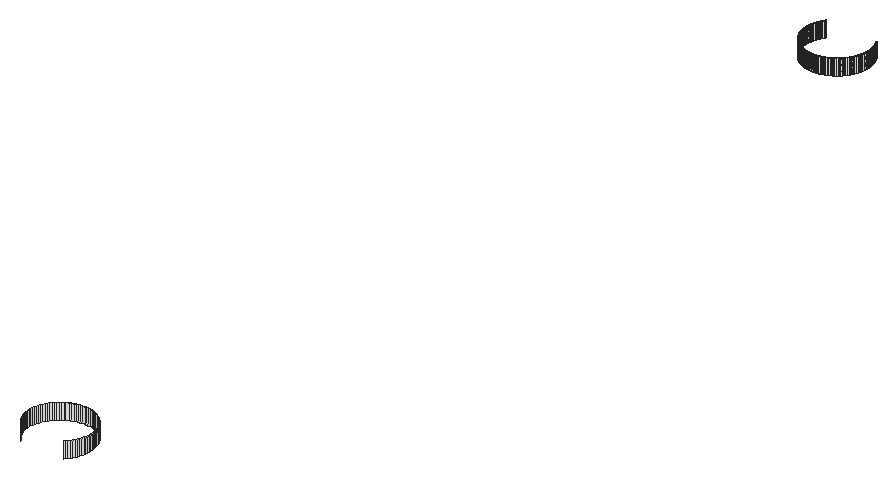
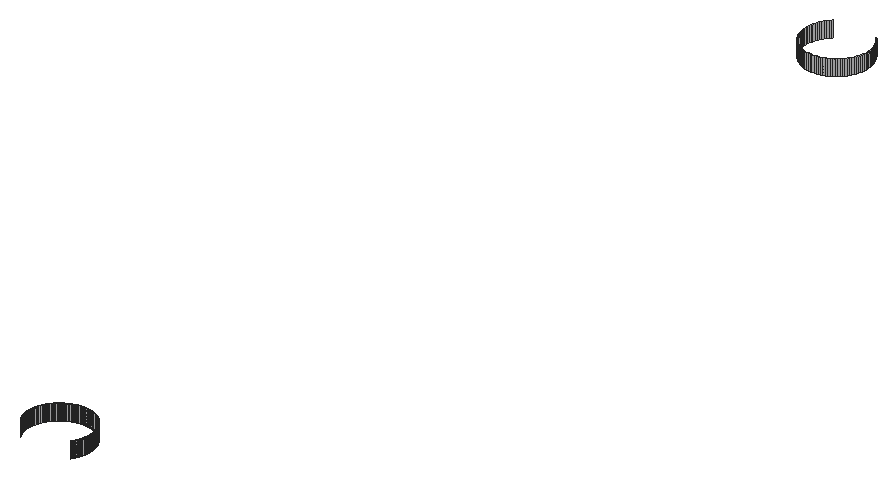
# SketchUp Ruby script. Lengths in inches.
U = 1.inch
M = Sketchup.active_model
def pt(a) = Geom::Point3d.new(a.map { |v| v * U })
def face(e, loops, mat)
  f = e.add_face(loops[0].map { |a| pt(a) })
  loops[1..].each { |l| e.add_face(l.map { |a| pt(a) }).erase! }
  f.material = f.back_material = mat if mat
  f
end
# faces: each face lists its corners as indices into pts; further lists are holes
def faces(e, pts, list, mat = nil) = list.each { |f| face(e, (f[0].is_a?(Array) ? f : [f]).map { |l| l.map { |i| pts[i] } }, mat) }
# xy, xz, yz: faces in a plane at the given z, y or x. An outline is a flat list of corners, or four numbers for a rectangle; further outlines are holes
def ring(l) = l.size == 4 ? [[l[0], l[1]], [l[2], l[1]], [l[2], l[3]], [l[0], l[3]]] : l.each_slice(2).to_a
def flat(e, list, mat, &to3) = list.each { |f| face(e, (f[0].is_a?(Array) ? f : [f]).map { |l| ring(l).map { |u, v| to3.(u, v) } }, mat) }
def xy(e, z, list, mat = nil) = flat(e, list, mat) { |x, y| [x, y, z] }
def xz(e, y, list, mat = nil) = flat(e, list, mat) { |x, z| [x, y, z] }
def yz(e, x, list, mat = nil) = flat(e, list, mat) { |y, z| [x, y, z] }
def lines(e, pts, list) = list.each { |a, b| e.add_line(pt(pts[a]), pt(pts[b])) }
# prism: a flat outline (further loops are holes) pulled along v
def prism(e, loops, v, mat = nil)
  f = face(e, loops, mat); d = Geom::Vector3d.new(v.map { |x| x * U })
  f.pushpull(f.normal.samedirection?(d) ? d.length : -d.length)
end
def box(e, o, s, mat = nil) = prism(e, [[o, [o[0] + s[0], o[1], o[2]], [o[0] + s[0], o[1] + s[1], o[2]], [o[0], o[1] + s[1], o[2]]]], [0, 0, s[2]], mat)
def at(x, y, z, deg = 0) = Geom::Transformation.translation(pt([x, y, z])) * Geom::Transformation.rotation(ORIGIN, Z_AXIS, deg.degrees)
def axes(o, x, y, z) = Geom::Transformation.new([*x, 0, *y, 0, *z, 0, *pt(o).to_a, 1])
def part(name) = M.definitions.add(name)
# library, detail: a bought-in or finely detailed component or shape, given as its bounding box
def library(name, o, s) = part(name).tap { |d| box(d.entities, o, s) }
def detail(e, o, s) = box(e.add_group.entities, o, s)
def put(e, d, t, mat = nil) = e.add_instance(d, t).tap { |i| i.material = mat if mat }
def group(e, t, mat = nil) = e.add_group.tap { |g| g.transformation = t; g.material = mat if mat }.entities
root = M.entities
M.materials.add("[Quartz Light Grey]").color = [251, 251, 252]
xz(root,170.71,[[32.98,111.81,33.1,112.81]],"[Quartz Light Grey]")
xz(root,222.0625,[[38.98,111.81,39,112.81],[39,111.81,39.02,112.81]],"[Quartz Light Grey]")
xz(root,222.07,[[38.8125,111.81,38.85,112.81],[38.85,111.81,38.875,112.81],[38.875,111.81,38.9,112.81],[39.1,111.81,39.125,112.81],[39.125,111.81,39.15,112.81],
  [39.15,111.81,39.1875,112.81]],"[Quartz Light Grey]")
xz(root,222.08,[[38.73,111.81,38.75,112.81],[38.75,111.81,38.77,112.81],[39.23,111.81,39.25,112.81],[39.25,111.81,39.27,112.81]],"[Quartz Light Grey]")
xz(root,222.09,[[38.65,111.81,38.6875,112.81],[39.3125,111.81,39.35,112.81]],"[Quartz Light Grey]")
xz(root,222.1,[[38.6,111.81,38.625,112.81],[39.375,111.81,39.4,112.81]],"[Quartz Light Grey]")
xz(root,222.2,[[38.26,111.81,38.28,112.81],[39.72,111.81,39.74,112.81]],"[Quartz Light Grey]")
yz(root,31,[[168.6875,111.81,168.8125,112.81]],"[Quartz Light Grey]")
yz(root,35,[[168.6,111.81,168.73,112.81]],"[Quartz Light Grey]")
yz(root,37,[[223.9375,111.81,223.96,112.81],[223.96,111.81,224,112.81],[224,111.81,224.04,112.81],[224.04,111.81,224.0625,112.81],[224.0625,111.81,224.08,112.81],
  [224.08,111.81,224.125,112.81],[224.125,111.81,224.17,112.81],[224.17,111.81,224.1875,112.81]],"[Quartz Light Grey]")
yz(root,37.01,[[223.83,111.81,223.875,112.81],[223.875,111.81,223.92,112.81],[224.21,111.81,224.25,112.81],[224.25,111.81,224.29,112.81]],"[Quartz Light Grey]")
yz(root,37.02,[[223.79,111.81,223.8125,112.81],[224.3125,111.81,224.33,112.81]],"[Quartz Light Grey]")
yz(root,37.03,[[223.71,111.81,223.75,112.81],[224.375,111.81,224.42,112.81]],"[Quartz Light Grey]")
yz(root,37.04,[[223.67,111.81,223.6875,112.81],[224.4375,111.81,224.46,112.81]],"[Quartz Light Grey]")
yz(root,37.1,[[223.42,111.81,223.44,112.81],[224.68,111.81,224.7,112.81]],"[Quartz Light Grey]")
yz(root,40.9,[[223.42,111.81,223.44,112.81],[224.68,111.81,224.7,112.81]],"[Quartz Light Grey]")
yz(root,40.96,[[223.67,111.81,223.6875,112.81],[224.4375,111.81,224.46,112.81]],"[Quartz Light Grey]")
yz(root,40.97,[[223.71,111.81,223.75,112.81],[224.375,111.81,224.42,112.81]],"[Quartz Light Grey]")
yz(root,40.98,[[223.79,111.81,223.8125,112.81],[224.3125,111.81,224.33,112.81]],"[Quartz Light Grey]")
yz(root,40.99,[[223.83,111.81,223.875,112.81],[223.875,111.81,223.92,112.81],[224.21,111.81,224.25,112.81],[224.25,111.81,224.29,112.81]],"[Quartz Light Grey]")
yz(root,41,[[223.9375,111.81,223.96,112.81],[223.96,111.81,224,112.81],[224,111.81,224.04,112.81],[224.04,111.81,224.0625,112.81],[224.0625,111.81,224.08,112.81],
  [224.08,111.81,224.125,112.81],[224.125,111.81,224.17,112.81],[224.17,111.81,224.1875,112.81]],"[Quartz Light Grey]")
p = [[31.56,167.32,111.81],[31.47,167.42,111.81],[31.47,167.42,112.81],[31.56,167.32,112.81],[34.47,167.36,111.81],[34.38,167.27,111.81],
  [34.38,167.27,112.81],[34.47,167.36,112.81],[31.39,167.52,111.81],[31.39,167.52,112.81],[34.55,167.45,111.81],[34.55,167.45,112.81],
  [31.32,167.62,111.81],[31.32,167.62,112.81],[34.63,167.55,111.81],[34.63,167.55,112.81],[31.26,167.73,111.81],[31.26,167.73,112.81],
  [34.7,167.66,111.81],[34.7,167.66,112.81],[31.2,167.84,111.81],[31.2,167.84,112.81],[34.76,167.76,111.81],[34.76,167.76,112.81],
  [31.15,167.95,111.81],[31.15,167.95,112.81],[34.82,167.875,111.81],[34.82,167.875,112.81],[34.87,167.99,111.81],[34.87,167.99,112.81],
  [31.1,168.07,111.81],[31.1,168.07,112.81],[34.91,168.11,111.81],[34.91,168.11,112.81],[31.07,168.19,111.81],[31.07,168.19,112.81],
  [34.94,168.23,111.81],[34.94,168.23,112.81],[31.04,168.3125,111.81],[31.04,168.3125,112.81],[34.97,168.35,111.81],[34.97,168.35,112.81],
  [31.02,168.4375,111.81],[31.02,168.4375,112.81],[31.01,168.5625,111.81],[31.01,168.5625,112.81],[34.99,168.48,111.81],[34.99,168.48,112.81],
  [35,168.6,111.81],[35,168.6,112.81],[31,168.6875,111.81],[31,168.6875,112.81],[34.99,168.86,111.81],[35,168.73,111.81],
  [35,168.73,112.81],[34.99,168.86,112.81],[31,168.8125,111.81],[31.01,168.9375,111.81],[31.01,168.9375,112.81],[31,168.8125,112.81],
  [31.03,169.0625,111.81],[31.03,169.0625,112.81],[34.98,168.98,111.81],[34.98,168.98,112.81],[34.96,169.1,111.81],[34.96,169.1,112.81],
  [31.06,169.19,111.81],[31.06,169.19,112.81],[34.93,169.23,111.81],[34.93,169.23,112.81],[31.09,169.31,111.81],[31.09,169.31,112.81],
  [34.9,169.35,111.81],[34.9,169.35,112.81],[31.13,169.42,111.81],[31.13,169.42,112.81],[34.85,169.46,111.81],[34.85,169.46,112.81],
  [31.18,169.54,111.81],[31.18,169.54,112.81],[31.24,169.65,111.81],[31.24,169.65,112.81],[34.8,169.58,111.81],[34.8,169.58,112.81],
  [34.74,169.69,111.81],[34.74,169.69,112.81],[31.3,169.76,111.81],[31.3,169.76,112.81],[34.68,169.8,111.81],[34.68,169.8,112.81],
  [31.37,169.87,111.81],[31.37,169.87,112.81],[34.61,169.9,111.81],[34.61,169.9,112.81],[31.45,169.97,111.81],[31.45,169.97,112.81],
  [34.53,170,111.81],[34.53,170,112.81],[31.53,170.0625,111.81],[31.53,170.0625,112.81],[34.44,170.09,111.81],[34.44,170.09,112.81],
  [31.62,170.15,111.81],[31.62,170.15,112.81],[34.35,170.18,111.81],[34.35,170.18,112.81],[31.71,170.24,111.81],[31.71,170.24,112.81],
  [31.81,170.3125,111.81],[31.81,170.3125,112.81],[34.26,170.26,111.81],[34.26,170.26,112.81],[31.91,170.39,111.81],[31.91,170.39,112.81],
  [34.05,170.41,111.81],[34.16,170.34,111.81],[34.16,170.34,112.81],[34.05,170.41,112.81],[32.02,170.45,111.81],[32.02,170.45,112.81],
  [33.94,170.47,111.81],[33.94,170.47,112.81],[32.13,170.51,111.81],[32.13,170.51,112.81],[32.24,170.56,111.81],[32.24,170.56,112.81],
  [33.72,170.58,111.81],[33.83,170.53,111.81],[33.83,170.53,112.81],[33.72,170.58,112.81],[32.36,170.6,111.81],[32.36,170.6,112.81],
  [32.48,170.64,111.81],[32.48,170.64,112.81],[32.6,170.67,111.81],[32.6,170.67,112.81],[33.48,170.65,111.81],[33.6,170.62,111.81],
  [33.6,170.62,112.81],[33.48,170.65,112.81],[32.73,170.69,111.81],[32.73,170.69,112.81],[32.85,170.7,111.81],[32.85,170.7,112.81],
  [32.98,170.71,111.81],[32.98,170.71,112.81],[33.1,170.71,111.81],[33.23,170.7,111.81],[33.23,170.7,112.81],[33.1,170.71,112.81],
  [33.35,170.68,111.81],[33.35,170.68,112.81],[38.48,222.13,111.81],[38.44,222.14,111.81],[38.44,222.14,112.81],[38.48,222.13,112.81],
  [38.4,222.15,111.81],[38.4,222.15,112.81],[38.5625,222.11,111.81],[38.52,222.12,111.81],[38.52,222.12,112.81],[38.5625,222.11,112.81],
  [38.5,222.125,111.81],[38.5,222.125,112.81],[38.65,222.09,111.81],[38.625,222.1,111.81],[38.625,222.1,112.81],[38.65,222.09,112.81],
  [38.6,222.1,111.81],[38.6,222.1,112.81],[38.73,222.08,111.81],[38.6875,222.09,111.81],[38.6875,222.09,112.81],[38.73,222.08,112.81],
  [38.8125,222.07,111.81],[38.77,222.08,111.81],[38.77,222.08,112.81],[38.8125,222.07,112.81],[38.98,222.0625,111.81],[38.9375,222.06,111.81],
  [38.9375,222.06,112.81],[38.98,222.0625,112.81],[38.9,222.07,111.81],[38.9,222.07,112.81],[39.0625,222.06,111.81],[39.02,222.0625,111.81],
  [39.02,222.0625,112.81],[39.0625,222.06,112.81],[39.1,222.07,111.81],[39.1,222.07,112.81],[39.23,222.08,111.81],[39.1875,222.07,111.81],
  [39.1875,222.07,112.81],[39.23,222.08,112.81],[39.3125,222.09,111.81],[39.27,222.08,111.81],[39.27,222.08,112.81],[39.3125,222.09,112.81],
  [39.375,222.1,111.81],[39.35,222.09,111.81],[39.35,222.09,112.81],[39.375,222.1,112.81],[39.4375,222.11,111.81],[39.4,222.1,111.81],
  [39.4,222.1,112.81],[39.4375,222.11,112.81],[39.48,222.12,111.81],[39.48,222.12,112.81],[39.5,222.125,111.81],[39.5,222.125,112.81],
  [39.52,222.13,111.81],[39.52,222.13,112.81],[39.56,222.14,111.81],[39.56,222.14,112.81],[39.6,222.15,111.81],[39.6,222.15,112.81],
  [38.17,222.24,111.81],[38.15,222.25,111.81],[38.15,222.25,112.81],[38.17,222.24,112.81],[38.26,222.2,111.81],[38.24,222.21,111.81],
  [38.24,222.21,112.81],[38.26,222.2,112.81],[38.21,222.23,111.81],[38.21,222.23,112.81],[38.36,222.17,111.81],[38.32,222.18,111.81],
  [38.32,222.18,112.81],[38.36,222.17,112.81],[38.28,222.2,111.81],[38.28,222.2,112.81],[38.38,222.16,111.81],[38.38,222.16,112.81],
  [39.62,222.16,111.81],[39.62,222.16,112.81],[39.64,222.17,111.81],[39.64,222.17,112.81],[39.68,222.18,111.81],[39.68,222.18,112.81],
  [39.72,222.2,111.81],[39.72,222.2,112.81],[39.76,222.21,111.81],[39.74,222.2,111.81],[39.74,222.2,112.81],[39.76,222.21,112.81],
  [39.79,222.23,111.81],[39.79,222.23,112.81],[39.83,222.24,111.81],[39.83,222.24,112.81],[39.85,222.25,111.81],[39.85,222.25,112.81],
  [37.98,222.34,111.81],[37.95,222.36,111.81],[37.95,222.36,112.81],[37.98,222.34,112.81],[38.06,222.3,111.81],[38.04,222.3125,111.81],
  [38.04,222.3125,112.81],[38.06,222.3,112.81],[38.02,222.32,111.81],[38.02,222.32,112.81],[38.13,222.26,111.81],[38.13,222.26,112.81],
  [38.09,222.28,111.81],[38.09,222.28,112.81],[39.87,222.26,111.81],[39.87,222.26,112.81],[39.91,222.28,111.81],[39.91,222.28,112.81],
  [39.94,222.3,111.81],[39.94,222.3,112.81],[39.96,222.3125,111.81],[39.96,222.3125,112.81],[39.98,222.32,111.81],[39.98,222.32,112.81],
  [40.02,222.34,111.81],[40.02,222.34,112.81],[40.05,222.36,111.81],[40.05,222.36,112.81],[37.875,222.41,111.81],[37.84,222.43,111.81],
  [37.84,222.43,112.81],[37.875,222.41,112.81],[37.82,222.45,111.81],[37.82,222.45,112.81],[37.81,222.46,111.81],[37.81,222.46,112.81],
  [37.93,222.375,111.81],[37.93,222.375,112.81],[37.91,222.39,111.81],[37.91,222.39,112.81],[40.07,222.375,111.81],[40.07,222.375,112.81],
  [40.09,222.39,111.81],[40.09,222.39,112.81],[40.125,222.41,111.81],[40.125,222.41,112.81],[40.16,222.43,111.81],[40.16,222.43,112.81],
  [40.18,222.45,111.81],[40.18,222.45,112.81],[40.19,222.46,111.81],[40.19,222.46,112.81],[37.77,222.48,111.81],[37.74,222.51,111.81],
  [37.74,222.51,112.81],[37.77,222.48,112.81],[37.73,222.52,111.81],[37.73,222.52,112.81],[37.71,222.54,111.81],[37.71,222.54,112.81],
  [37.68,222.5625,111.81],[37.68,222.5625,112.81],[40.23,222.48,111.81],[40.23,222.48,112.81],[40.26,222.51,111.81],[40.26,222.51,112.81],
  [40.27,222.52,111.81],[40.27,222.52,112.81],[40.29,222.54,111.81],[40.29,222.54,112.81],[40.32,222.5625,111.81],[40.32,222.5625,112.81],
  [37.65,222.59,111.81],[37.65,222.59,112.81],[37.63,222.61,111.81],[37.63,222.61,112.81],[37.62,222.62,111.81],[37.62,222.62,112.81],
  [37.59,222.65,111.81],[37.59,222.65,112.81],[37.56,222.68,111.81],[37.56,222.68,112.81],[40.35,222.59,111.81],[40.35,222.59,112.81],
  [40.37,222.61,111.81],[40.37,222.61,112.81],[40.38,222.62,111.81],[40.38,222.62,112.81],[40.41,222.65,111.81],[40.41,222.65,112.81],
  [40.44,222.68,111.81],[40.44,222.68,112.81],[37.54,222.69,111.81],[37.54,222.69,112.81],[37.53,222.71,111.81],[37.53,222.71,112.81],
  [37.5,222.74,111.81],[37.5,222.74,112.81],[37.47,222.77,111.81],[37.47,222.77,112.81],[40.46,222.69,111.81],[40.46,222.69,112.81],
  [40.47,222.71,111.81],[40.47,222.71,112.81],[40.5,222.74,111.81],[40.5,222.74,112.81],[40.53,222.77,111.81],[40.53,222.77,112.81],
  [37.46,222.79,111.81],[37.45,222.8,111.81],[37.45,222.8,112.81],[37.46,222.79,112.81],[37.42,222.84,111.81],[37.42,222.84,112.81],
  [37.39,222.87,111.81],[37.39,222.87,112.81],[40.54,222.79,111.81],[40.54,222.79,112.81],[40.55,222.8,111.81],[40.55,222.8,112.81],
  [40.58,222.84,111.81],[40.58,222.84,112.81],[40.61,222.87,111.81],[40.61,222.87,112.81],[37.37,222.9,111.81],[37.35,222.9375,111.81],
  [37.35,222.9375,112.81],[37.37,222.9,112.81],[37.32,222.97,111.81],[37.32,222.97,112.81],[37.38,222.89,111.81],[37.38,222.89,112.81],
  [40.62,222.89,111.81],[40.62,222.89,112.81],[40.63,222.9,111.81],[40.63,222.9,112.81],[40.65,222.9375,111.81],[40.65,222.9375,112.81],
  [40.68,222.97,111.81],[40.68,222.97,112.81],[37.3125,222.99,111.81],[37.3125,222.99,112.81],[37.3,223.01,111.81],[37.3,223.01,112.81],
  [37.28,223.05,111.81],[37.28,223.05,112.81],[37.26,223.08,111.81],[37.26,223.08,112.81],[40.6875,222.99,111.81],[40.6875,222.99,112.81],
  [40.7,223.01,111.81],[40.7,223.01,112.81],[40.72,223.05,111.81],[40.72,223.05,112.81],[40.74,223.08,111.81],[40.74,223.08,112.81],
  [37.25,223.1,111.81],[37.25,223.1,112.81],[37.24,223.12,111.81],[37.24,223.12,112.81],[37.22,223.16,111.81],[37.22,223.16,112.81],
  [40.75,223.1,111.81],[40.75,223.1,112.81],[40.76,223.12,111.81],[40.76,223.12,112.81],[40.78,223.16,111.81],[40.78,223.16,112.81],
  [37.2,223.19,111.81],[37.2,223.19,112.81],[37.19,223.21,111.81],[37.19,223.21,112.81],[37.18,223.23,111.81],[37.18,223.23,112.81],
  [37.17,223.27,111.81],[37.17,223.27,112.81],[40.8,223.19,111.81],[40.8,223.19,112.81],[40.81,223.21,111.81],[40.81,223.21,112.81],
  [40.82,223.23,111.81],[40.82,223.23,112.81],[40.83,223.27,111.81],[40.83,223.27,112.81],[37.15,223.31,111.81],[37.15,223.31,112.81],
  [37.14,223.33,111.81],[37.14,223.33,112.81],[37.13,223.35,111.81],[37.13,223.35,112.81],[37.12,223.39,111.81],[37.12,223.39,112.81],
  [40.85,223.31,111.81],[40.85,223.31,112.81],[40.86,223.33,111.81],[40.86,223.33,112.81],[40.87,223.35,111.81],[40.87,223.35,112.81],
  [40.88,223.39,111.81],[40.88,223.39,112.81],[37.1,223.42,111.81],[37.1,223.42,112.81],[37.1,223.44,111.81],[37.09,223.47,111.81],
  [37.09,223.47,112.81],[37.1,223.44,112.81],[40.9,223.42,111.81],[40.9,223.42,112.81],[40.91,223.47,111.81],[40.9,223.44,111.81],
  [40.9,223.44,112.81],[40.91,223.47,112.81],[37.08,223.51,111.81],[37.08,223.51,112.81],[37.07,223.54,111.81],[37.07,223.54,112.81],
  [37.0625,223.57,111.81],[37.0625,223.57,112.81],[40.92,223.51,111.81],[40.92,223.51,112.81],[40.93,223.54,111.81],[40.93,223.54,112.81],
  [40.9375,223.57,111.81],[40.9375,223.57,112.81],[37.06,223.59,111.81],[37.05,223.625,111.81],[37.05,223.625,112.81],[37.06,223.59,112.81],
  [37.04,223.67,111.81],[37.04,223.67,112.81],[40.94,223.59,111.81],[40.94,223.59,112.81],[40.95,223.625,111.81],[40.95,223.625,112.81],
  [40.96,223.67,111.81],[40.96,223.67,112.81],[37.04,223.6875,111.81],[37.03,223.71,111.81],[37.03,223.71,112.81],[37.04,223.6875,112.81],
  [40.97,223.71,111.81],[40.96,223.6875,111.81],[40.96,223.6875,112.81],[40.97,223.71,112.81],[37.03,223.75,111.81],[37.02,223.79,111.81],
  [37.02,223.79,112.81],[37.03,223.75,112.81],[37.02,223.8125,111.81],[37.01,223.83,111.81],[37.01,223.83,112.81],[37.02,223.8125,112.81],
  [40.98,223.79,111.81],[40.97,223.75,111.81],[40.97,223.75,112.81],[40.98,223.79,112.81],[40.99,223.83,111.81],[40.98,223.8125,111.81],
  [40.98,223.8125,112.81],[40.99,223.83,112.81],[37.01,223.92,111.81],[37,223.9375,111.81],[37,223.9375,112.81],[37.01,223.92,112.81],
  [41,223.9375,111.81],[40.99,223.92,111.81],[40.99,223.92,112.81],[41,223.9375,112.81],[37,224.1875,111.81],[37.01,224.21,111.81],
  [37.01,224.21,112.81],[37,224.1875,112.81],[40.99,224.21,111.81],[41,224.1875,111.81],[41,224.1875,112.81],[40.99,224.21,112.81],
  [37.01,224.29,111.81],[37.02,224.3125,111.81],[37.02,224.3125,112.81],[37.01,224.29,112.81],[37.02,224.33,111.81],[37.03,224.375,111.81],
  [37.03,224.375,112.81],[37.02,224.33,112.81],[40.98,224.3125,111.81],[40.99,224.29,111.81],[40.99,224.29,112.81],[40.98,224.3125,112.81],
  [40.97,224.375,111.81],[40.98,224.33,111.81],[40.98,224.33,112.81],[40.97,224.375,112.81],[37.03,224.42,111.81],[37.04,224.4375,111.81],
  [37.04,224.4375,112.81],[37.03,224.42,112.81],[40.96,224.4375,111.81],[40.97,224.42,111.81],[40.97,224.42,112.81],[40.96,224.4375,112.81],
  [37.04,224.46,111.81],[37.05,224.5,111.81],[37.05,224.5,112.81],[37.04,224.46,112.81],[37.06,224.54,111.81],[37.06,224.54,112.81],
  [37.0625,224.56,111.81],[37.0625,224.56,112.81],[40.94,224.54,111.81],[40.95,224.5,111.81],[40.95,224.5,112.81],[40.94,224.54,112.81],
  [40.9375,224.56,111.81],[40.9375,224.56,112.81],[40.96,224.46,111.81],[40.96,224.46,112.81],[37.07,224.58,111.81],[37.07,224.58,112.81],
  [37.08,224.62,111.81],[37.08,224.62,112.81],[37.09,224.66,111.81],[37.09,224.66,112.81],[40.93,224.58,111.81],[40.93,224.58,112.81],
  [40.92,224.62,111.81],[40.92,224.62,112.81],[40.91,224.66,111.81],[40.91,224.66,112.81],[37.1,224.68,111.81],[37.1,224.68,112.81],
  [37.1,224.7,111.81],[37.12,224.74,111.81],[37.12,224.74,112.81],[37.1,224.7,112.81],[37.13,224.78,111.81],[37.13,224.78,112.81],
  [40.9,224.68,111.81],[40.9,224.68,112.81],[40.88,224.74,111.81],[40.9,224.7,111.81],[40.9,224.7,112.81],[40.88,224.74,112.81],
  [40.87,224.78,111.81],[40.87,224.78,112.81],[37.14,224.8,111.81],[37.14,224.8,112.81],[37.15,224.82,111.81],[37.15,224.82,112.81],
  [37.17,224.86,111.81],[37.17,224.86,112.81],[40.83,224.86,111.81],[40.85,224.82,111.81],[40.85,224.82,112.81],[40.83,224.86,112.81],
  [40.86,224.8,111.81],[40.86,224.8,112.81],[37.18,224.89,111.81],[37.18,224.89,112.81],[37.19,224.91,111.81],[37.19,224.91,112.81],
  [37.2,224.93,111.81],[37.2,224.93,112.81],[37.22,224.97,111.81],[37.22,224.97,112.81],[40.82,224.89,111.81],[40.82,224.89,112.81],
  [40.81,224.91,111.81],[40.81,224.91,112.81],[40.8,224.93,111.81],[40.8,224.93,112.81],[40.78,224.97,111.81],[40.78,224.97,112.81],
  [37.24,225.01,111.81],[37.24,225.01,112.81],[37.25,225.03,111.81],[37.25,225.03,112.81],[37.26,225.05,111.81],[37.26,225.05,112.81],
  [37.28,225.08,111.81],[37.28,225.08,112.81],[40.74,225.05,111.81],[40.75,225.03,111.81],[40.75,225.03,112.81],[40.74,225.05,112.81],
  [40.76,225.01,111.81],[40.76,225.01,112.81],[37.3,225.12,111.81],[37.3,225.12,112.81],[37.3125,225.13,111.81],[37.3125,225.13,112.81],
  [37.32,225.15,111.81],[37.32,225.15,112.81],[37.35,225.1875,111.81],[37.35,225.1875,112.81]]
faces(root,p,[[0,1,2,3],[4,5,6,7],[1,8,9,2],[10,4,7,11],[8,12,13,9],[14,10,11,15],[12,16,17,13],[18,14,15,19],
  [16,20,21,17],[22,18,19,23],[20,24,25,21],[26,22,23,27],[28,26,27,29],[24,30,31,25],[32,28,29,33],[30,34,35,31],
  [36,32,33,37],[34,38,39,35],[40,36,37,41],[38,42,43,39],[42,44,45,43],[46,40,41,47],[48,46,47,49],[44,50,51,45],
  [52,53,54,55],[56,57,58,59],[57,60,61,58],[62,52,55,63],[64,62,63,65],[60,66,67,61],[68,64,65,69],[66,70,71,67],
  [72,68,69,73],[70,74,75,71],[76,72,73,77],[74,78,79,75],[78,80,81,79],[82,76,77,83],[84,82,83,85],[80,86,87,81],
  [88,84,85,89],[86,90,91,87],[92,88,89,93],[90,94,95,91],[96,92,93,97],[94,98,99,95],[100,96,97,101],[98,102,103,99],
  [104,100,101,105],[102,106,107,103],[106,108,109,107],[110,104,105,111],[108,112,113,109],[114,115,116,117],[115,110,111,116],[112,118,119,113],
  [120,114,117,121],[118,122,123,119],[122,124,125,123],[126,127,128,129],[127,120,121,128],[124,130,131,125],[130,132,133,131],[132,134,135,133],
  [136,137,138,139],[137,126,129,138],[134,140,141,135],[140,142,143,141],[142,144,145,143],[146,147,148,149],[147,150,151,148],[150,136,139,151],
  [152,153,154,155],[153,156,157,154],[158,159,160,161],[159,162,163,160],[162,152,155,163],[164,165,166,167],[168,158,161,169],[170,171,172,173],
  [174,175,176,177],[178,179,180,181],[179,182,183,180],[184,185,186,187],[188,184,187,189],[190,191,192,193],[194,195,196,197],[198,199,200,201],
  [202,203,204,205],[206,202,205,207],[208,206,207,209],[210,208,209,211],[212,210,211,213],[214,212,213,215],[216,217,218,219],[220,221,222,223],
  [221,224,225,222],[224,216,219,225],[226,227,228,229],[227,230,231,228],[156,232,233,157],[232,226,229,233],[234,214,215,235],[236,234,235,237],
  [238,236,237,239],[240,238,239,241],[242,243,244,245],[246,242,245,247],[248,246,247,249],[250,248,249,251],[252,253,254,255],[256,257,258,259],
  [257,260,261,258],[260,252,255,261],[217,262,263,218],[262,264,265,263],[264,256,259,265],[266,250,251,267],[268,266,267,269],[270,268,269,271],
  [272,270,271,273],[274,272,273,275],[276,274,275,277],[278,276,277,279],[280,281,282,283],[281,284,285,282],[284,286,287,285],[253,288,289,254],
  [288,290,291,289],[290,280,283,291],[292,278,279,293],[294,292,293,295],[296,294,295,297],[298,296,297,299],[300,298,299,301],[302,300,301,303],
  [304,305,306,307],[305,308,309,306],[308,310,311,309],[310,312,313,311],[286,304,307,287],[314,302,303,315],[316,314,315,317],[318,316,317,319],
  [320,318,319,321],[322,320,321,323],[312,324,325,313],[324,326,327,325],[326,328,329,327],[328,330,331,329],[330,332,333,331],[334,322,323,335],
  [336,334,335,337],[338,336,337,339],[340,338,339,341],[342,340,341,343],[332,344,345,333],[344,346,347,345],[346,348,349,347],[348,350,351,349],
  [352,342,343,353],[354,352,353,355],[356,354,355,357],[358,356,357,359],[360,361,362,363],[361,364,365,362],[364,366,367,365],[350,360,363,351],
  [368,358,359,369],[370,368,369,371],[372,370,371,373],[374,372,373,375],[376,377,378,379],[377,380,381,378],[366,382,383,367],[382,376,379,383],
  [384,374,375,385],[386,384,385,387],[388,386,387,389],[390,388,389,391],[380,392,393,381],[392,394,395,393],[394,396,397,395],[396,398,399,397],
  [400,390,391,401],[402,400,401,403],[404,402,403,405],[406,404,405,407],[398,408,409,399],[408,410,411,409],[410,412,413,411],[414,406,407,415],
  [416,414,415,417],[418,416,417,419],[412,420,421,413],[420,422,423,421],[422,424,425,423],[424,426,427,425],[428,418,419,429],[430,428,429,431],
  [432,430,431,433],[434,432,433,435],[426,436,437,427],[436,438,439,437],[438,440,441,439],[440,442,443,441],[444,434,435,445],[446,444,445,447],
  [448,446,447,449],[450,448,449,451],[442,452,453,443],[454,455,456,457],[458,450,451,459],[460,461,462,463],[455,464,465,456],[464,466,467,465],
  [466,468,469,467],[470,460,463,471],[472,470,471,473],[474,472,473,475],[476,477,478,479],[477,480,481,478],[468,476,479,469],[482,474,475,483],
  [484,482,483,485],[486,484,485,487],[488,489,490,491],[492,493,494,495],[496,497,498,499],[500,501,502,503],[504,505,506,507],[508,509,510,511],
  [512,513,514,515],[516,517,518,519],[520,521,522,523],[524,525,526,527],[528,529,530,531],[532,533,534,535],[536,537,538,539],[540,541,542,543],
  [544,545,546,547],[548,549,550,551],[552,553,554,555],[553,556,557,554],[556,558,559,557],[560,561,562,563],[564,560,563,565],[561,566,567,562],
  [558,568,569,559],[568,570,571,569],[570,572,573,571],[574,564,565,575],[576,574,575,577],[578,576,577,579],[572,580,581,573],[582,583,584,585],
  [583,586,587,584],[588,578,579,589],[590,591,592,593],[594,590,593,595],[586,596,597,587],[596,598,599,597],[598,600,601,599],[602,603,604,605],
  [606,594,595,607],[603,606,607,604],[600,608,609,601],[608,610,611,609],[610,612,613,611],[612,614,615,613],[616,602,605,617],[618,616,617,619],
  [620,618,619,621],[622,620,621,623],[614,624,625,615],[624,626,627,625],[626,628,629,627],[628,630,631,629],[632,633,634,635],[636,622,623,637],
  [633,636,637,634],[630,638,639,631],[638,640,641,639],[640,642,643,641],[642,644,645,643]],"[Quartz Light Grey]")
